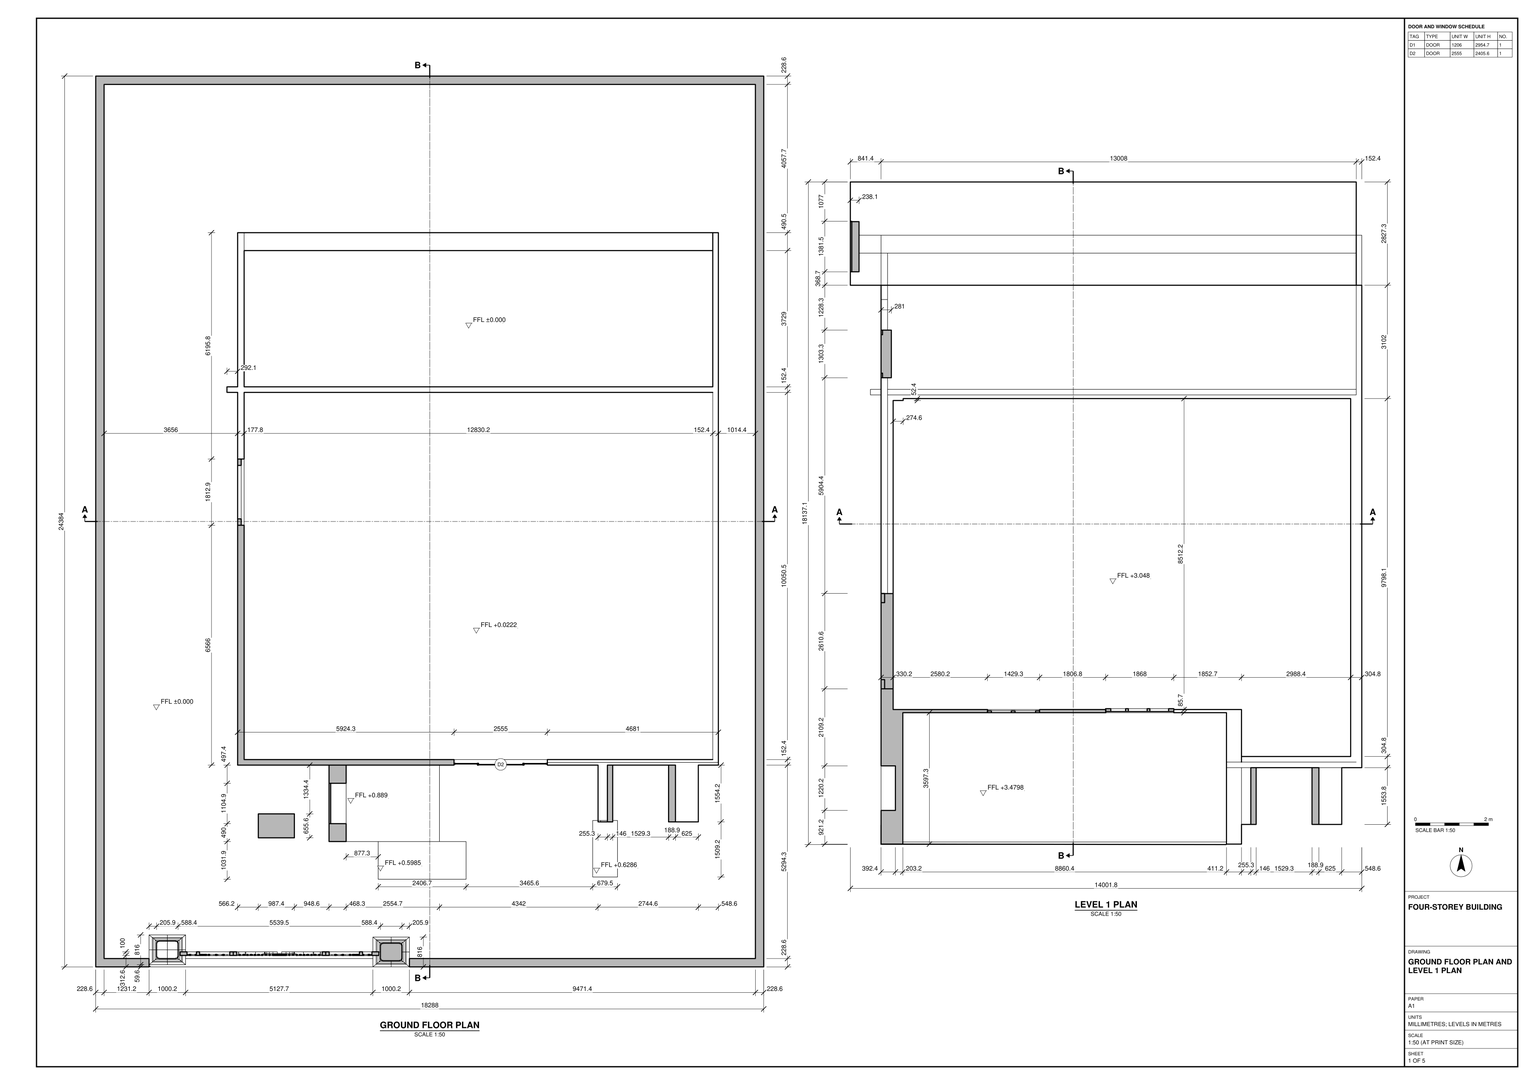
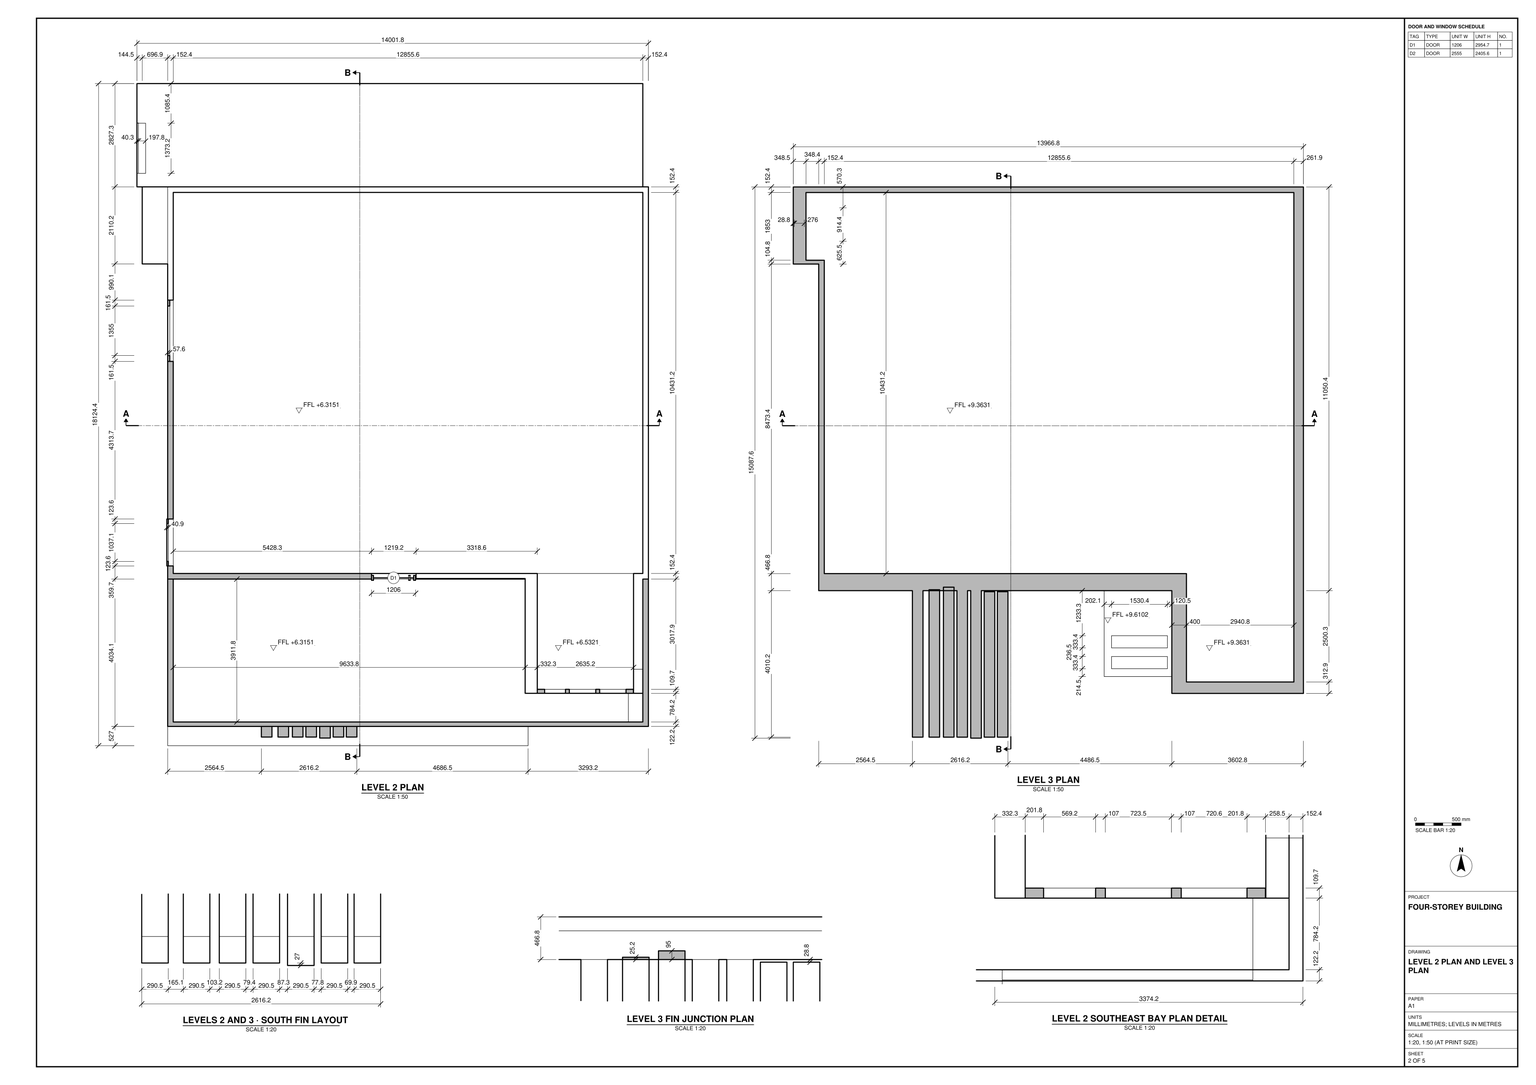
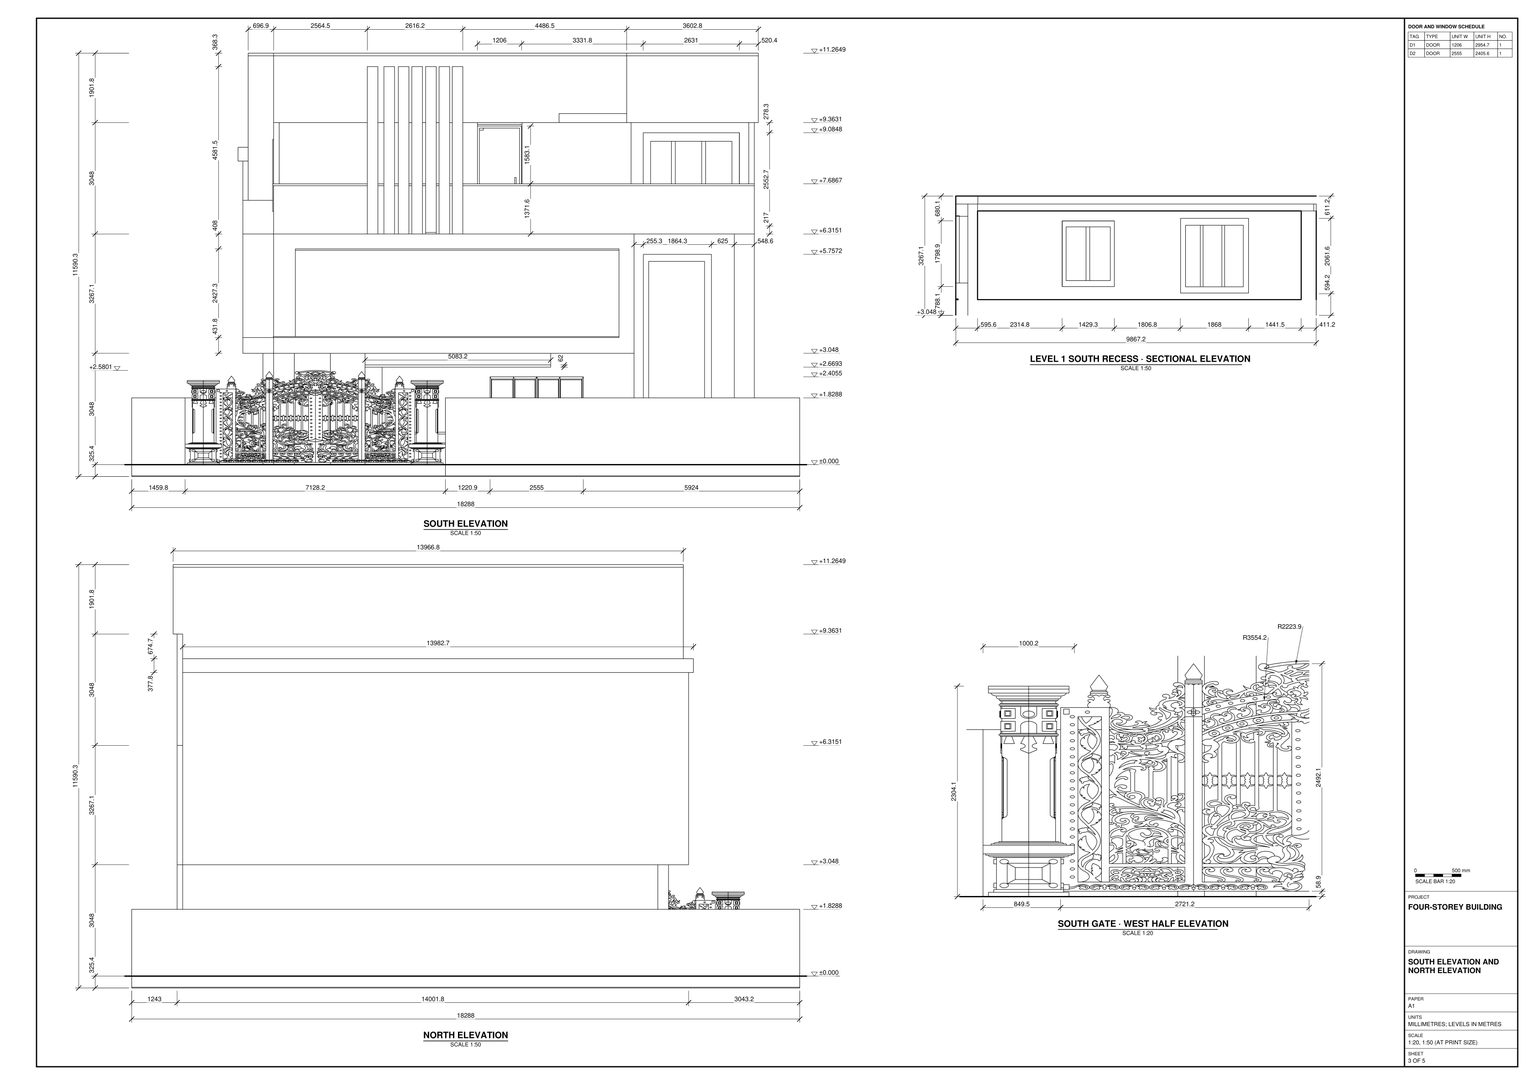
Build the four-storey building and its enclosed site in SketchUp from task_files/diagram_01.pdf. Work in millimetres. The complete model, including the site, measures 18288 mm east–west, 24384 mm north–south and 11590.3 mm from bottom to top. Set the ground floor at 0 mm and the successive storey levels at +3048 mm, +6315.1 mm and +9363.1 mm. Keep the local changes in slab height shown on the plans distinct from these storey levels.

Set out the perimeter wall, the gate and its flanking piers on the south boundary. Position the building within the enclosure using the setbacks on the ground-floor plan. Follow the wall thicknesses and slab edges on each plan rather than repeating one footprint through all four storeys. Model the flat roof and parapets, the projecting bays, and the doors and windows in their drawn openings. Use the sectional elevation to place the windows behind the frame of the Level 1 south recess. Above it, use the plan details to set out the vertical fins and the glazed southeast bay.

Keep shell elements such as walls, slabs and roof, and each furniture or joinery piece shown, in separate groups or components. Use components for repeated parts. Decor and loose items may be any suitable library components. Save one SketchUp model as output_files/four_storey_building_and_its_gated_enclosure.skp.

# SketchUp Ruby script. Lengths in millimetres.
U = 1.mm
M = Sketchup.active_model
def pt(a) = Geom::Point3d.new(a.map { |v| v * U })
def face(e, loops, mat)
  f = e.add_face(loops[0].map { |a| pt(a) })
  loops[1..].each { |l| e.add_face(l.map { |a| pt(a) }).erase! }
  f.material = f.back_material = mat if mat
  f
end
# faces: each face lists its corners as indices into pts; further lists are holes
def faces(e, pts, list, mat = nil) = list.each { |f| face(e, (f[0].is_a?(Array) ? f : [f]).map { |l| l.map { |i| pts[i] } }, mat) }
# xy, xz, yz: faces in a plane at the given z, y or x. An outline is a flat list of corners, or four numbers for a rectangle; further outlines are holes
def ring(l) = l.size == 4 ? [[l[0], l[1]], [l[2], l[1]], [l[2], l[3]], [l[0], l[3]]] : l.each_slice(2).to_a
def flat(e, list, mat, &to3) = list.each { |f| face(e, (f[0].is_a?(Array) ? f : [f]).map { |l| ring(l).map { |u, v| to3.(u, v) } }, mat) }
def xy(e, z, list, mat = nil) = flat(e, list, mat) { |x, y| [x, y, z] }
def xz(e, y, list, mat = nil) = flat(e, list, mat) { |x, z| [x, y, z] }
def yz(e, x, list, mat = nil) = flat(e, list, mat) { |y, z| [x, y, z] }
def lines(e, pts, list) = list.each { |a, b| e.add_line(pt(pts[a]), pt(pts[b])) }
# prism: a flat outline (further loops are holes) pulled along v
def prism(e, loops, v, mat = nil)
  f = face(e, loops, mat); d = Geom::Vector3d.new(v.map { |x| x * U })
  f.pushpull(f.normal.samedirection?(d) ? d.length : -d.length)
end
def box(e, o, s, mat = nil) = prism(e, [[o, [o[0] + s[0], o[1], o[2]], [o[0] + s[0], o[1] + s[1], o[2]], [o[0], o[1] + s[1], o[2]]]], [0, 0, s[2]], mat)
def at(x, y, z, deg = 0) = Geom::Transformation.translation(pt([x, y, z])) * Geom::Transformation.rotation(ORIGIN, Z_AXIS, deg.degrees)
def axes(o, x, y, z) = Geom::Transformation.new([*x, 0, *y, 0, *z, 0, *pt(o).to_a, 1])
def part(name) = M.definitions.add(name)
# library, detail: a bought-in or finely detailed component or shape, given as its bounding box
def library(name, o, s) = part(name).tap { |d| box(d.entities, o, s) }
def detail(e, o, s) = box(e.add_group.entities, o, s)
def put(e, d, t, mat = nil) = e.add_instance(d, t).tap { |i| i.material = mat if mat }
def group(e, t, mat = nil) = e.add_group.tap { |g| g.transformation = t; g.material = mat if mat }.entities
root = M.entities
M.materials.add("[0128_White]").color = [255, 255, 255]
M.materials.add("[Color C08]").color = [102, 51, 0]
M.materials.add("[Color D02]").color = [255, 229, 153]
M.materials.add("[Color M04]").color = [188, 188, 188]
M.materials.add("[Color M06]").color = [86, 86, 86]
M.materials.add("[Color M07]").color = [58, 58, 58]
M.materials.add("[Color M07]1").color = [58, 58, 58]
M.materials.add("[Concrete Scored Jointless]").color = [140, 133, 127]
M.materials.add("[Metal_Corrogated_Shiny]").color = [193, 193, 193]
M.materials.add("[Translucent Glass Blue]").color = [100, 149, 237]
M.materials["[Translucent Glass Blue]"].alpha = 0.5
M.materials.add("[Translucent Glass Gray]").color = [128, 128, 128]
M.materials["[Translucent Glass Gray]"].alpha = 0.5
M.materials.add("[Wood Fence with Lattice]").color = [170, 106, 61]
M.materials.add("[Wood OSB]").color = [240, 195, 122]
M.materials.add("[Wood Veneer 01]").color = [120, 70, 37]
c1 = part("Component\#1")
box(c1.entities,[0,0,0],[8,40,80],"[Metal_Corrogated_Shiny]")
c2 = part("Door pull handle")
prism(c2.entities,[[[0,30,890],[0,30,900],[50,30,900],[50,30,0],[0,30,0],[0,30,10],[40,30,10],[40,30,890]]],[0,-30,0],"[Color M07]")
c3 = part("Framed glass door")
g1 = group(c3.entities,at(41,40,0))
g2 = group(g1,at(-46,0,0))
g3 = group(g2,at(45,0,0))
p = [[15,0,2060],[15,820,2060]]
lines(g3,p,[[0,1]])
g4 = group(g3,at(15,0,0))
yz(g4,0,[[0,0,820,2060]],"[Translucent Glass Gray]")
g5 = group(g2,at(-48.3,0,0))
put(g5,c1,axes([104.3,0,2060],[1,0,0],[0,0,-1],[0,1,0]))
put(g5,c1,axes([104.3,0,40],[1,0,0],[0,0,-1],[0,1,0]))
g6 = group(g2,at(0,720,200))
put(g6,c2,axes([60,0,0],[-1,0,0],[0,1,0],[0,0,1]))
put(g6,c2,at(60,0,0))
g7 = group(c3.entities,at(105,0,0))
g8 = group(g7,at(-100,0,0))
prism(g8,[[[100,860,0],[100,900,0],[100,900,2100],[100,0,2100],[100,0,0],[100,40,0],[100,40,2060],[100,860,2060]]],[-100,0,0],"[Metal_Corrogated_Shiny]")
c4 = part("door glass")
put(c4.entities,c3,at(0,105,0,-90))
c5 = library("20170416 - Larg Glass Door",[-30,0,0],[170,4000,2000])
c6 = library("Gate pier",[0,0,0],[850,850,3692.5])
c7 = library("Drawing1.dwg",[3859.7,90,-250],[4440,3834.1,108])
c8 = part("cổng")
p = [[0,0,0],[25.4,0,0],[492,0,0],[25.4,25.4,0]]
lines(c8.entities,p,[[0,1],[1,2],[1,3],[3,0]])
put(c8.entities,c6,axes([0,59.6,0.7],[0.96,0,0],[0,0.96,0],[0,0,0.96]),"[0128_White]")
put(c8.entities,c6,axes([4999.3,0,0],[0.96,0,0],[0,0.96,0],[0,0,0.96]),"[0128_White]")
put(c8.entities,c7,axes([-3166.7,162.6,0.7],[1,0,0],[0,0,1],[0,-1,0]),"[Color M04]")
g9 = group(c8.entities,at(2510.2,307.6,3835.3),"[Color M07]1")
prism(g9,[[[36.5,5,67.1],[0,5,7.2],[51.1,5,24.7],[108.8,5,44.6],[166.3,5,60.6],[224.7,5,73.1],[283.7,5,82.1],[343.2,5,87.5],[402.9,5,89.3],[462.5,5,87.5],[522,5,82.1],[581,5,73.1],[639.4,5,60.6],[696.9,5,44.6],[754.7,5,24.7],[826.5,5,0],[769.2,5,67.1],[710.2,5,87.4],[650.1,5,104.1],[589.1,5,117.2],[527.4,5,126.5],[465.2,5,132.2],[402.9,5,134.1],[340.5,5,132.2],[278.3,5,126.5],[216.6,5,117.2],[155.6,5,104.1],[95.5,5,87.4]]],[0,25,0])
c9 = part("Group\#1")
xy(c9.entities,0,[[0,0,152.4,862]])
xy(c9.entities,83,[[0,83,152.4,779]],"[Color C08]")
xy(c9.entities,779,[[0,83,152.4,779]],"[Color C08]")
xy(c9.entities,862,[[0,0,152.4,862]],"[Color C08]")
xz(c9.entities,0,[[0,0,152.4,862]],"[Color C08]")
xz(c9.entities,83,[[0,83,152.4,779]],"[Color C08]")
xz(c9.entities,779,[[0,83,152.4,779]],"[Color C08]")
xz(c9.entities,862,[[0,0,152.4,862]],"[Color C08]")
yz(c9.entities,0,[[[0,0,862,862],[83,83,779,779]]],"[Color C08]")
yz(c9.entities,0,[[83,83,779,779]],"[Translucent Glass Gray]")
yz(c9.entities,152.4,[[[0,0,862,862],[83,83,779,779]]],"[Color C08]")
c10 = part("Group\#2")
xy(c10.entities,0,[[0,0,3233.7,152.4]])
xy(c10.entities,248.1,[[1480.7,0,1712.7,152.4]])
xy(c10.entities,248.1,[[248.1,0,1480.7,152.4],[1712.7,0,2985.7,152.4]],"[Color C08]")
xy(c10.entities,2469.7,[[248.1,0,1480.7,152.4],[1480.7,0,1712.7,152.4],[1712.7,0,2985.7,152.4]])
xy(c10.entities,2717.8,[[0,0,3233.7,152.4]],"[Color C08]")
xz(c10.entities,0,[[[0,0,3233.7,2717.8],[248.1,248.1,2985.7,2469.7]],[1480.7,248.1,1712.7,2469.7]],"[Color C08]")
xz(c10.entities,0,[[248.1,248.1,1480.7,2469.7],[1712.7,248.1,2985.7,2469.7]],"[Translucent Glass Gray]")
xz(c10.entities,152.4,[[[0,0,3233.7,2717.8],[248.1,248.1,2985.7,2469.7]],[1480.7,248.1,1712.7,2469.7]],"[Color C08]")
yz(c10.entities,0,[[0,0,152.4,2717.8]],"[Color C08]")
yz(c10.entities,248.1,[[0,248.1,152.4,2469.7]],"[Color C08]")
yz(c10.entities,1480.7,[[0,248.1,152.4,2469.7]],"[Color C08]")
yz(c10.entities,1712.7,[[0,248.1,152.4,2469.7]],"[Color C08]")
yz(c10.entities,2985.7,[[0,248.1,152.4,2469.7]],"[Color C08]")
yz(c10.entities,3233.7,[[0,0,152.4,2717.8]],"[Color C08]")
c11 = part("Group\#3")
xy(c11.entities,0,[[0,0,3233.7,152.4]])
xy(c11.entities,248.1,[[947.7,0,1079.2,152.4],[1968.5,0,2100,152.4]])
xy(c11.entities,248.1,[[248.1,0,947.7,152.4],[1079.2,0,1968.5,152.4],[2100,0,2985.7,152.4]],"[Color C08]")
xy(c11.entities,2469.7,[[248.1,0,947.7,152.4],[947.7,0,1079.2,152.4],[1079.2,0,1968.5,152.4],[1968.5,0,2100,152.4],[2100,0,2985.7,152.4]])
xy(c11.entities,2717.8,[[0,0,3233.7,152.4]],"[Color C08]")
xz(c11.entities,0,[[[0,0,3233.7,2717.8],[248.1,248.1,2985.7,2469.7]],[947.7,248.1,1079.2,2469.7],[1968.5,248.1,2100,2469.7]],"[Color C08]")
xz(c11.entities,0,[[248.1,248.1,947.7,2469.7],[1079.2,248.1,1968.5,2469.7],[2100,248.1,2985.7,2469.7]],"[Translucent Glass Gray]")
xz(c11.entities,152.4,[[[0,0,3233.7,2717.8],[248.1,248.1,2985.7,2469.7]],[947.7,248.1,1079.2,2469.7],[1968.5,248.1,2100,2469.7]],"[Color C08]")
yz(c11.entities,0,[[0,0,152.4,2717.8]],"[Color C08]")
yz(c11.entities,248.1,[[0,248.1,152.4,2469.7]],"[Color C08]")
yz(c11.entities,947.7,[[0,248.1,152.4,2469.7]],"[Color C08]")
yz(c11.entities,1079.2,[[0,248.1,152.4,2469.7]],"[Color C08]")
yz(c11.entities,1968.5,[[0,248.1,152.4,2469.7]],"[Color C08]")
yz(c11.entities,2100,[[0,248.1,152.4,2469.7]],"[Color C08]")
yz(c11.entities,2985.7,[[0,248.1,152.4,2469.7]],"[Color C08]")
yz(c11.entities,3233.7,[[0,0,152.4,2717.8]],"[Color C08]")
xy(root,-20.6,[[0,0,18288,24384]])
xy(root,0,[[0,0,18288,24384]])
xy(root,304.8,[[1459.8,0,8588,228.6],[6386.8,3430.6,9409.8,5522.9],[15871.3,3968.7,16496.3,3968.7,16496.3,5522.9,17045,5522.9,17045,5597.5,12363.9,5597.5,12363.9,5522.9,13751.8,5522.9,13751.8,4007.4,14007,4007.4,14007,5522.9,15871.3,5522.9],[13751.8,3968.7,13821.3,4007.4],[15682.4,3968.7,15871.3,5522.9],
  [14007,4007.4,14153.1,5522.9],[5844.3,5522.9,8644.6,5522.9,8644.6,5597.5,9808.9,5597.5,9808.9,5675.3,4062.4,5675.3,4062.4,15725.8,16892.6,15725.8,16892.6,5675.3,12363.9,5675.3,12363.9,5597.5,17045,5597.5,17045,20097.7,16892.6,20097.7,16892.6,15878.2,4062.4,15878.2,4062.4,20097.7,3884.6,20097.7,3884.6,15878.2,3592.5,15878.2,3592.5,15725.8,3884.6,15725.8,3884.6,5597.5,5844.3,5597.5],[3884.6,5522.9,5844.3,5597.5],[8644.6,5522.9,9808.9,5597.5],[4062.4,15878.2,16892.6,19607.2],
  [4062.4,19607.2,16892.6,20097.7]])
xy(root,304.8,[[[228.6,228.6,18059.4,24155.4],[7732.5,2398.7,7732.5,3430.6,6386.8,3430.6,6386.8,5522.9,3884.6,5522.9,3884.6,15725.8,3592.5,15725.8,3592.5,15878.2,3884.6,15878.2,3884.6,20097.7,17045,20097.7,17045,5522.9,16496.3,5522.9,16496.3,3968.7,15682.4,3968.7,15682.4,5522.9,14153.1,5522.9,14153.1,4007.4,14284.1,4007.4,14284.1,2459.6,13604.7,2459.6,13604.7,4007.4,13751.8,4007.4,13751.8,5522.9,12363.9,5522.9,12363.9,5675.3,9808.9,5675.3,9808.9,5522.9,9409.8,5522.9,9409.8,3430.6,10139.1,3430.6,10139.1,2398.7],[4450.8,3532.8,5438.2,4188.5]]],"[Concrete Scored Jointless]")
xy(root,304.8,[[0,0,0,24384,18288,24384,18288,0,8588,0,8588,228.6,18059.4,228.6,18059.4,24155.4,228.6,24155.4,228.6,228.6,1459.8,228.6,1459.8,0]],"[Wood Fence with Lattice]")
xy(root,327,[[4062.4,5675.3,16892.6,15725.8]])
xy(root,858.8,[[7732.5,2398.7,10139.1,3430.6],[13604.7,2459.6,13604.7,4007.4,13751.8,4007.4,13751.8,3968.7,13821.3,3968.7,13821.3,4007.4,14284.1,4007.4,14284.1,2459.6]])
xy(root,903.3,[[7732.5,2398.7,10139.1,3430.6]],"[Color M06]")
xy(root,933.4,[[13821.3,3968.7,14007,4007.4],[14007,3968.7,14153.1,4007.4]])
xy(root,933.4,[[13604.7,2459.6,14284.1,2459.6,14284.1,4007.4,14153.1,4007.4,14153.1,3968.7,13751.8,3968.7,13751.8,4007.4,13604.7,4007.4]],"[Color M06]")
xy(root,1143,[[6386.8,3430.6,9409.8,5522.9]])
xy(root,1193.8,[[6386.8,3430.6,6855.1,5522.9]])
xy(root,1193.8,[[6855.1,3430.6,9409.8,5522.9]],"[Color M06]")
xy(root,1197.6,[[3884.6,12089,4062.4,13901.9]])
xy(root,1449.5,[[6386.8,3920.6,6855.1,5025.5]])
xy(root,2133.6,[[0,0,1459.8,0,1459.8,228.6,228.6,228.6,228.6,24155.4,18059.4,24155.4,18059.4,228.6,8588,228.6,8588,0,18288,0,18288,24384,0,24384]],"[Wood Fence with Lattice]")
xy(root,2225,[[3884.6,7579.3,4062.4,8200],[3884.6,8890.5,4062.4,9511.3]])
xy(root,2603.6,[[6386.8,3920.6,6855.1,5025.5]])
xy(root,2710.4,[[9808.9,5522.9,12363.9,5597.5],[9808.9,5597.5,12363.9,5675.3]])
xy(root,2885.1,[[3884.6,12089,4062.4,13901.9]])
xy(root,2952,[[3884.6,7579.3,4062.4,8200],[3884.6,8890.5,4062.4,9511.3]])
xy(root,2974.1,[[6386.8,3430.6,6855.1,3743.8],[6855.1,3430.6,11470,3743.8],[6386.8,3743.8,6855.1,5522.9]])
xy(root,3352.8,[[3884.6,3430.6,6386.8,5522.9],[6386.8,3430.6,6855.1,5522.9],[6855.1,3430.6,11470,3743.8],[4450.8,3532.8,5438.2,4188.5],[13751.8,5827.7,16740.2,5827.7,16740.2,15625.8,4489.5,15625.8,4489.5,15573.4,4214.8,15573.4,4214.8,7113.6,13751.8,7113.6],
  [3592.5,15725.8,3884.6,15878.2],[4062.4,15725.8,16892.6,15878.2],[4062.4,15878.2,16892.6,18727.7],[3884.6,18337.2,4062.4,18727.7],[3043.2,18727.7,3884.6,19607.2],
  [3884.6,18727.7,4062.4,19607.2],[16892.6,18727.7,17045,20097.7],[3043.2,19607.2,3884.6,20097.7],[3884.6,19607.2,16892.6,20097.7],[3043.2,20097.7,16892.6,21555]])
xy(root,3352.8,[[11470,3430.6,11470,3743.8,6855.1,3743.8,6855.1,5522.9,13751.8,5522.9,13751.8,3430.6]],"[Color M06]")
xy(root,3784.6,[[3884.6,3417.9,13340.6,3430.6],[3884.6,3430.6,3884.6,7027.9,3946.9,7027.9,3946.9,3488.3,13340.6,3488.3,13340.6,3430.6],[4480.2,3488.3,13340.6,7027.9],[3884.6,7027.9,3946.9,8570.9]])
xy(root,3797.3,[[3884.6,3954.9,3946.9,4215.3],[3884.6,4215.3,3946.9,5927.6],[3884.6,5927.6,3946.9,7027.9]])
xy(root,3810,[[3875.1,3417.9,13340.6,3417.9,4480.2,3430.6,3884.6,3430.6,3884.6,3954.9,3875.1,3954.9],[13340.6,3417.9,13340.6,3488.3,4480.2,3488.3,4480.2,3430.6],[3884.6,3430.6,3946.9,3954.9],[3946.9,3430.6,4480.2,3488.3],[3884.6,7027.9,3946.9,8570.9]])
xy(root,3964,[[10038.6,7027.9,11899.1,7113.6]])
xy(root,4140.9,[[6800.3,7027.9,8224.3,7113.6]])
xy(root,4238.9,[[3884.6,7681.2,4214.8,10287.8]])
xy(root,4311.6,[[3884.6,4351.8,4277,5572],[4277,4351.8,4287.9,5572]],"[Color D02]")
xy(root,4374.6,[[3043.2,19096.5,3281.4,20469.6]])
xy(root,4378.5,[[3884.6,16196.1,4165.6,17499.5]])
xy(root,5352.9,[[3884.6,14095.4,4214.8,14805]])
xy(root,5869.9,[[14153.1,3968.7,15682.4,5522.9]])
xy(root,5896.4,[[3884.6,4351.8,4277,5572]])
xy(root,5916.8,[[3884.6,16196.1,4165.6,17499.5]])
xy(root,5936.4,[[6800.3,7027.9,8224.3,7113.6]])
xy(root,6008.7,[[10038.6,7027.9,11899.1,7113.6]])
xy(root,6062,[[14007,3968.7,15871.3,5522.9]])
xy(root,6062.5,[[3884.6,14095.4,4214.8,14805]])
xy(root,6064.5,[[3884.6,7681.2,4214.8,10287.8]])
xy(root,6211.9,[[4480.2,3430.6,13340.6,7027.9],[13340.6,5827.7,13685.1,7027.9]])
xy(root,6400.8,[[13751.8,5827.7,13751.8,7113.6,4214.8,7113.6,4214.8,15573.4,16740.2,15573.4,16740.2,5827.7],[4489.5,15573.4,16740.2,15625.8]])
xy(root,6444.7,[[3043.2,19096.5,3281.4,20469.6]])
xy(root,6619.9,[[6449.1,3667.1,6739.6,3957.6],[6904.7,3667.1,7195.2,3957.6],[7298.4,3667.1,7588.9,3957.6],[7668.3,3667.1,7958.8,3957.6],[8046.1,3667.1,8336.6,3957.6],
  [8414.4,3667.1,8704.9,3957.6],[8774.8,3667.1,9065.3,3957.6],[3884.6,3957.6,3884.6,7991.7,4037,7991.7,4037,4079.9,13751.8,4079.9,13751.8,3957.6],[13751.8,3957.6,16496.3,3968.7],[16496.3,3957.6,16496.3,4079.9,16892.6,4079.9,16892.6,5522.9,17045,5522.9,17045,3957.6],
  [13751.8,3968.7,16496.3,4079.9],[4037,4079.9,16496.3,4079.9,16496.3,4864.1,13670.8,4864.1,13670.8,7991.7,4037,7991.7],[16496.3,4079.9,16892.6,4864.1],[13670.8,4864.1,13670.8,8006,10684.5,8006,10684.5,8144.1,16892.6,8144.1,16892.6,18575.3,4037,18575.3,4037,8144.1,9465.3,8144.1,9465.3,7991.7,3884.6,7991.7,3884.6,18727.7,17045,18727.7,17045,7991.7,16892.6,7991.7,16892.6,5522.9,16496.3,5522.9,16496.3,4864.1],[16496.3,4864.1,16892.6,5522.9],
  [16892.6,5522.9,17045,7991.7],[9465.3,7991.7,10684.5,8144.1],[10684.5,7991.7,13670.8,8006],[4037,8144.1,16892.6,18575.3]])
xy(root,6619.9,[[3884.6,3430.6,13751.8,3430.6,13751.8,3957.6,9065.3,3957.6,9065.3,3667.1,8774.8,3667.1,8774.8,3957.6,8704.9,3957.6,8704.9,3667.1,8414.4,3667.1,8414.4,3957.6,8336.6,3957.6,8336.6,3667.1,8046.1,3667.1,8046.1,3957.6,7958.8,3957.6,7958.8,3667.1,7668.3,3667.1,7668.3,3957.6,7588.9,3957.6,7588.9,3667.1,7298.4,3667.1,7298.4,3957.6,7195.2,3957.6,7195.2,3667.1,6904.7,3667.1,6904.7,3957.6,6739.6,3957.6,6739.6,3667.1,6449.1,3667.1,6449.1,3957.6,3884.6,3957.6]],"[Color M06]")
xy(root,6661.2,[[8046.1,3640.1,8336.6,3667.1],[8046.1,3667.1,8336.6,3957.6]])
xy(root,6836.9,[[14003.1,4864.1,16638.4,8144.1]])
xy(root,7233.2,[[3884.6,8351.5,4037,9635.7]])
xy(root,7540.6,[[3187.7,16617.5,3884.6,18727.7]])
xy(root,7553.7,[[3884.6,13949.5,4037,15627.5]])
xy(root,7940.7,[[3860.8,3937,3884.6,7991.7],[3884.6,3937,6449.1,3957.6],[3884.6,3957.6,3884.6,7991.7,4037,7991.7,4037,4079.9,16892.6,4079.9,16892.6,7991.7,17045,7991.7,17045,3957.6]])
xy(root,7991.5,[[3860.8,3937,6449.1,3937,6449.1,3957.6,3884.6,3957.6,3884.6,7991.7,3860.8,7991.7],[3884.6,3957.6,17045,3957.6,17045,7991.7,16892.6,7991.7,16892.6,4079.9,4037,4079.9,4037,7991.7,3884.6,7991.7]],"[Color M06]")
xy(root,8243.8,[[3187.7,17243,3492.5,18157.4]])
xy(root,8615.4,[[2909.9,18727.7,3043.2,21618.5],[3043.2,18727.7,16892.6,21555],[3043.2,21555,16892.6,21618.5]])
xy(root,8993.2,[[2909.9,18727.7,16892.6,21618.5]],"[Color M06]")
xy(root,9122.1,[[3884.6,13949.5,4037,15627.5]])
xy(root,9209.6,[[3884.6,8351.5,4037,9635.7]])
xy(root,9389.6,[[14003.1,4864.1,16638.4,8144.1]])
xy(root,9413.8,[[3187.7,17243,3492.5,18157.4]])
xy(root,9617.1,[[4037,8144.1,16892.6,18575.3]])
xy(root,9667.9,[[13551.8,4864.1,13670.8,5177.1],[16892.6,4864.1,17154.5,5177.1],[13951.8,5177.1,16892.6,5177.1,16892.6,18575.3,3536.2,18575.3,3536.2,16722.3,4037,16722.3,4037,8144.1,13951.8,8144.1],[13551.8,5177.1,13670.8,7677.4],[13670.8,5177.1,13951.8,7677.4],
  [16892.6,5177.1,17154.5,7677.4],[[11698.8,5326.3,11698.8,7677.4,10684.5,7677.4,10684.5,7991.7,13658.1,7991.7,13658.1,7677.4,13551.8,7677.4,13551.8,5326.3],[11900.9,6110.7,13431.3,6444.1],[11900.9,5540.8,13431.3,5874.1]],[3884.6,7677.4,4037,7991.7],[4037,7677.4,9465.3,7991.7],[9465.3,7677.4,10684.5,8144.1],
  [13658.1,7677.4,13670.8,7991.7],[13670.8,7677.4,13951.8,7991.7],[16892.6,7677.4,17154.5,7991.7],[10684.5,7991.7,13658.1,8006],[13658.1,7991.7,13670.8,8006],
  [13670.8,7991.7,13670.8,8006,13658.1,8006,13658.1,8144.1,13951.8,8144.1,13951.8,7991.7],[17045,7991.7,17154.5,18727.7]])
xy(root,9915,[[[11698.8,5326.3,13551.8,7677.4],[11900.9,5540.8,13431.3,5874.1],[11900.9,6110.7,13431.3,6444.1]]])
xy(root,10819.3,[[6449.1,3957.6,6739.6,7677.4],[6904.7,3957.6,7195.2,7702.5],[7298.4,3957.6,7588.9,7772.4],[7668.3,3957.6,7958.8,7677.4],[8046.1,3957.6,8336.6,7677.4],
  [8414.4,3957.6,8704.9,7648.6],[8774.8,3957.6,9065.3,7648.6]])
xy(root,11201.4,[[8046.1,3640.1,8336.6,7677.4],[6449.1,3667.1,6739.6,7677.4],[6904.7,3667.1,7195.2,7702.5],[7298.4,3667.1,7588.9,7772.4],[7668.3,3667.1,7958.8,7677.4],
  [8414.4,3667.1,8704.9,7648.6],[8774.8,3667.1,9065.3,7648.6]])
xy(root,11496.7,[[[13551.8,4864.1,13551.8,7677.4,3884.6,7677.4,3884.6,16617.5,3187.7,16617.5,3187.7,18727.7,17154.5,18727.7,17154.5,4864.1],[13951.8,5177.1,16892.6,5177.1,16892.6,18575.3,3536.2,18575.3,3536.2,16722.3,4037,16722.3,4037,8144.1,13951.8,8144.1]]])
xy(root,11569.7,[[[13551.8,4864.1,17154.5,4864.1,17154.5,18727.7,3187.7,18727.7,3187.7,16617.5,3884.6,16617.5,3884.6,7677.4,13551.8,7677.4],[13951.8,5177.1,13951.8,8144.1,4037,8144.1,4037,16722.3,3536.2,16722.3,3536.2,18575.3,16892.6,18575.3,16892.6,5177.1]]],"[Color M06]")
xz(root,0,[[0,-20.6,18288,0]])
xz(root,0,[[0,0,8588,304.8],[8588,0,18288,304.8],[0,304.8,1459.8,2133.6],[8588,304.8,18288,2133.6]],"[Wood Fence with Lattice]")
xz(root,228.6,[[228.6,304.8,1459.8,2133.6],[8588,304.8,18059.4,2133.6]],"[Wood Fence with Lattice]")
xz(root,2398.7,[[7732.5,858.8,10139.1,903.3]],"[Color M06]")
xz(root,2398.7,[[7732.5,304.8,10139.1,858.8]],"[Wood OSB]")
xz(root,2459.6,[[13604.7,858.8,14284.1,933.4]],"[Color M06]")
xz(root,2459.6,[[13604.7,304.8,14284.1,858.8]],"[Wood OSB]")
xz(root,3417.9,[[3875.1,3784.6,13340.6,3810]])
xz(root,3430.6,[[7732.5,304.8,9409.8,858.8],[9409.8,304.8,10139.1,858.8],[7732.5,858.8,9409.8,903.3],[9409.8,858.8,10139.1,903.3],[6386.8,1193.8,6855.1,2974.1]])
xz(root,3430.6,[[6386.8,1143,9409.8,1193.8],[6386.8,2974.1,11470,3036.1],[6386.8,3036.1,11470,3352.8],[3884.6,3352.8,13751.8,3352.8,13751.8,6619.9,3884.6,6619.9,3884.6,3810,4480.2,3810,4480.2,6211.9,13340.6,6211.9,13340.6,3784.6,3884.6,3784.6]],"[Color M06]")
xz(root,3430.6,[[6386.8,304.8,7732.5,304.8,7732.5,903.3,9409.8,903.3,9409.8,1143,6386.8,1143]],"[Wood OSB]")
xz(root,3488.3,[[3946.9,3784.6,4480.2,3810],[4480.2,3784.6,13340.6,3810]])
xz(root,3532.8,[[4450.8,304.8,5438.2,3352.8]],"[Color M06]")
xz(root,3640.1,[[8046.1,6661.2,8336.6,11201.4]])
xz(root,3667.1,[[6449.1,6619.9,6739.6,11201.4],[6904.7,6619.9,7195.2,11201.4],[7298.4,6619.9,7588.9,11201.4],[7668.3,6619.9,7958.8,11201.4],[8046.1,6619.9,8336.6,6661.2],
  [8414.4,6619.9,8704.9,11201.4],[8774.8,6619.9,9065.3,11201.4]])
xz(root,3743.8,[[6855.1,2974.1,11470,3352.8]],"[Color M06]")
xz(root,3920.6,[[6386.8,1449.5,6855.1,2603.6]])
xz(root,3937,[[3860.8,7940.7,6449.1,7991.5]],"[Color M06]")
xz(root,3954.9,[[3884.6,3797.3,3946.9,3810]])
xz(root,3957.6,[[6449.1,6619.9,6739.6,7940.7],[6739.6,6619.9,6904.7,7940.7],[6904.7,6619.9,7195.2,7940.7],[7195.2,6619.9,7298.4,7940.7],[7298.4,6619.9,7588.9,7940.7],
  [7588.9,6619.9,7668.3,7940.7],[7668.3,6619.9,7958.8,7940.7],[7958.8,6619.9,8046.1,7940.7],[8046.1,6619.9,8336.6,6661.2],[8336.6,6619.9,8414.4,7940.7],
  [8414.4,6619.9,8704.9,7940.7],[8704.9,6619.9,8774.8,7940.7],[8774.8,6619.9,9065.3,7940.7],[8046.1,6661.2,8336.6,7940.7],[3884.6,7940.7,6449.1,7991.5],
  [6449.1,7940.7,6739.6,7991.5],[6739.6,7940.7,6904.7,7991.5],[6904.7,7940.7,7195.2,7991.5],[7195.2,7940.7,7298.4,7991.5],[7298.4,7940.7,7588.9,7991.5],
  [7588.9,7940.7,7668.3,7991.5],[7668.3,7940.7,7958.8,7991.5],[7958.8,7940.7,8046.1,7991.5],[8046.1,7940.7,8336.6,7991.5],[8336.6,7940.7,8414.4,7991.5],
  [8414.4,7940.7,8704.9,7991.5],[8704.9,7940.7,8774.8,7991.5],[8774.8,7940.7,9065.3,7991.5],[6449.1,7991.5,6739.6,10819.3],[6904.7,7991.5,7195.2,10819.3],
  [7298.4,7991.5,7588.9,10819.3],[7668.3,7991.5,7958.8,10819.3],[8046.1,7991.5,8336.6,10819.3],[8414.4,7991.5,8704.9,10819.3],[8774.8,7991.5,9065.3,10819.3]])
xz(root,3957.6,[[9065.3,7940.7,17045,7991.5]],"[Color M06]")
xz(root,3957.6,[[3884.6,6619.9,6449.1,7940.7],[9065.3,6619.9,17045,7940.7]],"[Translucent Glass Blue]")
xz(root,3968.7,[[13751.8,304.8,13821.3,858.8],[15871.3,304.8,16496.3,304.8,16496.3,6619.9,13751.8,6619.9,13751.8,933.4,14007,933.4,14007,6062,15871.3,6062],[13751.8,858.8,13821.3,933.4]])
xz(root,3968.7,[[15682.4,304.8,15871.3,304.8,15871.3,6062,14007,6062,14007,933.4,14153.1,933.4,14153.1,5869.9,15682.4,5869.9]],"[Wood Veneer 01]")
xz(root,4007.4,[[13821.3,304.8,14007,858.8],[14007,304.8,14153.1,858.8],[13821.3,858.8,14007,933.4],[14007,858.8,14153.1,933.4]])
xz(root,4007.4,[[13604.7,858.8,13751.8,933.4],[14153.1,858.8,14284.1,933.4]],"[Color M06]")
xz(root,4007.4,[[13604.7,304.8,13751.8,858.8],[14153.1,304.8,14284.1,858.8]],"[Wood OSB]")
xz(root,4079.9,[[4037,7940.7,16892.6,7991.5]],"[Color M06]")
xz(root,4079.9,[[4037,6619.9,16892.6,7940.7]],"[Translucent Glass Blue]")
xz(root,4188.5,[[4450.8,304.8,5438.2,3352.8]],"[Color M06]")
xz(root,4351.8,[[3884.6,4311.6,4277,5896.4]],"[Color D02]")
xz(root,4864.1,[[[13670.8,6619.9,16892.6,9667.9],[14003.1,6836.9,16638.4,9389.6]],[13551.8,9667.9,17154.5,11496.7]])
xz(root,4864.1,[[13551.8,11496.7,17154.5,11569.7]],"[Color M06]")
xz(root,5025.5,[[6386.8,1449.5,6855.1,2603.6]])
xz(root,5177.1,[[13951.8,9667.9,16892.6,11496.7]])
xz(root,5177.1,[[13951.8,11496.7,16892.6,11569.7]],"[Color M06]")
xz(root,5326.3,[[11698.8,9667.9,13551.8,9915]])
xz(root,5522.9,[[3884.6,304.8,6386.8,3352.8],[6386.8,304.8,8644.6,1143],[9409.8,304.8,9808.9,304.8,9808.9,2710.4,12363.9,2710.4,12363.9,304.8,13751.8,304.8,13751.8,3352.8,6855.1,3352.8,6855.1,1193.8,9409.8,1193.8],[8644.6,304.8,9409.8,1143],[14007,304.8,14153.1,3352.8],
  [15682.4,304.8,15871.3,3352.8],[16496.3,304.8,17045,6619.9],[6386.8,1143,9409.8,1193.8],[6386.8,1193.8,6855.1,2974.1],[6386.8,2974.1,6855.1,3352.8],
  [14007,3352.8,14153.1,5869.9],[15682.4,3352.8,15871.3,5869.9],[14007,5869.9,15871.3,6062]])
xz(root,5522.9,[[14153.1,304.8,15682.4,5869.9]],"[Wood Veneer 01]")
xz(root,5540.8,[[11900.9,9667.9,13431.3,9915]])
xz(root,5572,[[3884.6,4311.6,4277,5896.4]],"[Color D02]")
xz(root,5675.3,[[4062.4,304.8,9808.9,327],[9808.9,304.8,12363.9,327],[12363.9,304.8,16892.6,327],[4062.4,327,4062.4,3352.8,16892.6,3352.8,16892.6,327,12363.9,327,12363.9,2710.4,9808.9,2710.4,9808.9,327]])
xz(root,5827.7,[[13751.8,3352.8,16740.2,6400.8],[13685.1,6211.9,13751.8,6400.8]])
xz(root,5874.1,[[11900.9,9667.9,13431.3,9915]])
xz(root,6110.7,[[11900.9,9667.9,13431.3,9915]])
xz(root,6444.1,[[11900.9,9667.9,13431.3,9915]])
xz(root,7027.9,[[3884.6,3784.6,3946.9,3797.3],[3884.6,3797.3,3946.9,3810],[4480.2,6211.9,13685.1,6400.8]])
xz(root,7027.9,[[[4480.2,3784.6,13340.6,6211.9],[10038.6,3964,11899.1,6008.7],[6800.3,4140.9,8224.3,5936.4]]],"[Color D02]")
xz(root,7113.6,[[[4214.8,3352.8,13751.8,6400.8],[10038.6,3964,11899.1,6008.7],[6800.3,4140.9,8224.3,5936.4]]])
xz(root,7579.3,[[3884.6,2225,4062.4,2952]])
xz(root,7648.6,[[8414.4,10819.3,8704.9,11201.4],[8774.8,10819.3,9065.3,11201.4]])
xz(root,7677.4,[[[3884.6,9667.9,11698.8,9667.9,11698.8,9915,13551.8,9915,13551.8,11496.7,3884.6,11496.7],[8046.1,10819.3,8336.6,11201.4],[6449.1,10819.3,6739.6,11201.4],[7668.3,10819.3,7958.8,11201.4]]])
xz(root,7677.4,[[3884.6,11496.7,13551.8,11569.7]],"[Color M06]")
xz(root,7681.2,[[3884.6,4238.9,4214.8,6064.5]])
xz(root,7702.5,[[6904.7,10819.3,7195.2,11201.4]])
xz(root,7772.4,[[7298.4,10819.3,7588.9,11201.4]])
xz(root,7991.7,[[3884.6,6619.9,4037,7940.7],[4037,6619.9,9465.3,9667.9],[10684.5,6619.9,13670.8,9667.9],[16892.6,6619.9,17045,7940.7],[3860.8,7940.7,3884.6,7991.5],
  [3884.6,7940.7,4037,7991.5],[16892.6,7940.7,17045,7991.5],[3884.6,7991.5,4037,9667.9],[16892.6,7991.5,17045,9667.9]])
xz(root,8006,[[10684.5,6619.9,13670.8,9667.9]])
xz(root,8144.1,[[4037,6619.9,9465.3,9617.1],[9465.3,6619.9,10684.5,9617.1],[[10684.5,6619.9,16892.6,9617.1],[14003.1,6836.9,16638.4,9389.6]],[4037,9617.1,9465.3,9667.9],[9465.3,9617.1,10684.5,9667.9],
  [4037,9667.9,13951.8,11496.7]])
xz(root,8144.1,[[4037,11496.7,13951.8,11569.7]],"[Color M06]")
xz(root,8200,[[3884.6,2225,4062.4,2952]])
xz(root,8351.5,[[3884.6,7233.2,4037,9209.6]])
xz(root,8570.9,[[3884.6,3784.6,3946.9,3810]])
xz(root,8890.5,[[3884.6,2225,4062.4,2952]])
xz(root,9511.3,[[3884.6,2225,4062.4,2952]])
xz(root,9635.7,[[3884.6,7233.2,4037,9209.6]])
xz(root,10287.8,[[3884.6,4238.9,4214.8,6064.5]])
xz(root,12089,[[3884.6,1197.6,4062.4,2885.1]])
xz(root,13901.9,[[3884.6,1197.6,4062.4,2885.1]])
xz(root,13949.5,[[3884.6,7553.7,4037,9122.1]])
xz(root,14095.4,[[3884.6,5352.9,4214.8,6062.5]])
xz(root,14805,[[3884.6,5352.9,4214.8,6062.5]])
xz(root,15573.4,[[4214.8,3352.8,4489.5,6400.8]])
xz(root,15625.8,[[4489.5,3352.8,16740.2,6400.8]])
xz(root,15627.5,[[3884.6,7553.7,4037,9122.1]])
xz(root,15725.8,[[3592.5,304.8,3884.6,3352.8],[4062.4,304.8,16892.6,327],[4062.4,327,16892.6,3352.8]])
xz(root,15878.2,[[3592.5,304.8,3884.6,1175.8],[4062.4,304.8,16892.6,3352.8],[3592.5,1175.8,3884.6,3352.8]])
xz(root,16196.1,[[3884.6,4378.5,4165.6,5916.8]])
xz(root,16617.5,[[3187.7,7540.6,3884.6,11496.7]])
xz(root,16617.5,[[3187.7,11496.7,3884.6,11569.7]],"[Color M06]")
xz(root,16722.3,[[3536.2,9667.9,4037,11496.7]])
xz(root,16722.3,[[3536.2,11496.7,4037,11569.7]],"[Color M06]")
xz(root,17243,[[3187.7,8243.8,3492.5,9413.8]])
xz(root,17499.5,[[3884.6,4378.5,4165.6,5916.8]])
xz(root,18157.4,[[3187.7,8243.8,3492.5,9413.8]])
xz(root,18575.3,[[4037,6619.9,4062.4,9617.1],[4062.4,6619.9,16892.6,9617.1],[4037,9617.1,4062.4,9667.9],[4062.4,9617.1,4398.1,9667.9],[4398.1,9617.1,4658.4,9667.9],
  [4658.4,9617.1,16892.6,9667.9],[3536.2,9667.9,16892.6,11496.7]])
xz(root,18575.3,[[3536.2,11496.7,16892.6,11569.7]],"[Color M06]")
xz(root,18727.7,[[3043.2,3352.8,3884.6,3784.6],[3884.6,3352.8,16892.6,6619.9],[16892.6,3352.8,17045,6619.9],[3043.2,3784.6,3884.6,6619.9],[3043.2,6619.9,3884.6,7540.6],
  [3884.6,6619.9,3884.6,7540.6,3187.7,7540.6,3187.7,8615.4,16892.6,8615.4,16892.6,6619.9],[16892.6,6619.9,17045,9667.9],[3043.2,7540.6,3187.7,8615.4],[2909.9,8615.4,3187.7,8993.2],[3187.7,8615.4,4062.4,8993.2],
  [4062.4,8615.4,16892.6,8993.2],[3187.7,8993.2,3187.7,11496.7,17154.5,11496.7,17154.5,9667.9,16892.6,9667.9,16892.6,8993.2]])
xz(root,18727.7,[[3187.7,11496.7,17154.5,11569.7]],"[Color M06]")
xz(root,19096.5,[[3043.2,4374.6,3281.4,6444.7]])
xz(root,19607.2,[[4062.4,304.8,16892.6,3352.8]])
xz(root,20097.7,[[3884.6,304.8,16892.6,3352.8],[16892.6,304.8,17045,3352.8]])
xz(root,20469.6,[[3043.2,4374.6,3281.4,6444.7]])
xz(root,21555,[[3043.2,3352.8,16892.6,8615.4]])
xz(root,21618.5,[[2909.9,8615.4,16892.6,8993.2]],"[Color M06]")
xz(root,24155.4,[[228.6,304.8,18059.4,2133.6]],"[Wood Fence with Lattice]")
xz(root,24384,[[0,-20.6,18288,0]])
xz(root,24384,[[0,0,18288,304.8],[0,304.8,18288,2133.6]],"[Wood Fence with Lattice]")
yz(root,0,[[0,-20.6,24384,0]])
yz(root,0,[[0,0,24384,304.8],[0,304.8,24384,2133.6]],"[Wood Fence with Lattice]")
yz(root,228.6,[[228.6,304.8,24155.4,2133.6]],"[Wood Fence with Lattice]")
yz(root,1459.8,[[0,304.8,228.6,2133.6]],"[Wood Fence with Lattice]")
yz(root,2909.9,[[18727.7,8615.4,21618.5,8993.2]],"[Color M06]")
yz(root,3043.2,[[[18727.7,3352.8,21555,8615.4],[19096.5,4374.6,20469.6,6444.7]]])
yz(root,3187.7,[[[16617.5,7540.6,18727.7,11496.7],[17243,8243.8,18157.4,9413.8]]])
yz(root,3187.7,[[16617.5,11496.7,18727.7,11569.7]],"[Color M06]")
yz(root,3281.4,[[19096.5,4374.6,20469.6,6444.7]])
yz(root,3492.5,[[17243,8243.8,18157.4,9413.8]])
yz(root,3536.2,[[16722.3,9667.9,18575.3,11496.7]])
yz(root,3536.2,[[16722.3,11496.7,18575.3,11569.7]],"[Color M06]")
yz(root,3592.5,[[15725.8,304.8,15878.2,3352.8]])
yz(root,3860.8,[[3937,7940.7,7991.7,7991.5]],"[Color M06]")
yz(root,3884.6,[[5522.9,304.8,5597.5,3352.8],[[5597.5,304.8,15725.8,3352.8],[12089,1197.6,13901.9,2885.1],[8890.5,2225,9511.3,2952],[7579.3,2225,8200,2952]],[15878.2,304.8,15878.2,1501.8,19607.2,1501.8,19607.2,3352.8,20097.7,3352.8,20097.7,304.8],[3430.6,3352.8,18727.7,3784.6],[3954.9,3784.6,7027.9,3797.3],
  [7027.9,3784.6,8182,3810],[8182,3784.6,8570.9,3810],[3957.6,7940.7,7991.7,7991.5],[7677.4,9667.9,16617.5,11496.7]])
yz(root,3884.6,[[[8570.9,3784.6,8570.9,3810,7027.9,3810,7027.9,3797.3,3954.9,3797.3,3954.9,3810,3430.6,3810,3430.6,6619.9,18727.7,6619.9,18727.7,3784.6],[7681.2,4238.9,10287.8,6064.5],[16196.1,4378.5,17499.5,5916.8],[4351.8,4311.6,5572,5896.4],[14095.4,5352.9,14805,6062.5]],[[7991.7,6619.9,7991.7,9667.9,16617.5,9667.9,16617.5,7540.6,18727.7,7540.6,18727.7,6619.9],[13949.5,7553.7,15627.5,9122.1],[8351.5,7233.2,9635.7,9209.6]],[7677.4,11496.7,16617.5,11569.7]],"[Color M06]")
yz(root,3884.6,[[3957.6,6619.9,7991.7,7940.7]],"[Translucent Glass Blue]")
yz(root,3884.6,[[15878.2,1501.8,19607.2,3352.8]],"[Translucent Glass Gray]")
yz(root,3946.9,[[5927.6,3765.6,7027.9,3784.6],[3488.3,3784.6,4215.3,3784.6,4215.3,3797.3,3954.9,3797.3,3954.9,3810,3488.3,3810],[4215.3,3784.6,5927.6,3797.3],[5927.6,3784.6,7027.9,3797.3],[7027.9,3784.6,8570.9,3810]])
yz(root,4037,[[[8144.1,6619.9,18575.3,9617.1],[13949.5,7553.7,15627.5,9122.1],[8351.5,7233.2,9635.7,9209.6]],[8144.1,9617.1,11462,9667.9],[11462,9617.1,11800.1,9667.9],[8144.1,9667.9,16722.3,11496.7]])
yz(root,4037,[[4079.9,7940.7,7991.7,7991.5],[8144.1,11496.7,16722.3,11569.7]],"[Color M06]")
yz(root,4037,[[4079.9,6619.9,7991.7,7940.7]],"[Translucent Glass Blue]")
yz(root,4062.4,[[5675.3,304.8,15725.8,327],[15878.2,304.8,19607.2,3352.8],[[5675.3,327,15725.8,3352.8],[12089,1197.6,13901.9,2885.1],[8890.5,2225,9511.3,2952],[7579.3,2225,8200,2952]]])
yz(root,4165.6,[[16196.1,4378.5,17499.5,5916.8]])
yz(root,4214.8,[[[7113.6,3352.8,15573.4,3352.8,15573.4,6400.8,7113.6,6400.8,7113.6,6064.5,10287.8,6064.5,10287.8,4238.9,7113.6,4238.9],[14095.4,5352.9,14805,6062.5]],[7113.6,4238.9,7681.2,6064.5],[7681.2,4238.9,10287.8,6064.5]])
yz(root,4277,[[4351.8,4311.6,5572,5896.4]],"[Color D02]")
yz(root,4450.8,[[3532.8,304.8,4188.5,3352.8]],"[Color M06]")
yz(root,4480.2,[[3488.3,3784.6,7027.9,3784.6,7027.9,6211.9,3430.6,6211.9,3430.6,3810,3488.3,3810]],"[Color D02]")
yz(root,4489.5,[[15573.4,3352.8,15625.8,6400.8]])
yz(root,5438.2,[[3532.8,304.8,4188.5,3352.8]],"[Color M06]")
yz(root,6386.8,[[[3430.6,1193.8,5522.9,2974.1],[3920.6,1449.5,5025.5,2603.6]]])
yz(root,6386.8,[[3430.6,1143,5522.9,1193.8],[3430.6,2974.1,5522.9,3036.1],[3430.6,3036.1,5522.9,3352.8]],"[Color M06]")
yz(root,6386.8,[[3430.6,304.8,5522.9,1143]],"[Wood OSB]")
yz(root,6449.1,[[3667.1,6619.9,3667.1,11201.4,7677.4,11201.4,7677.4,10819.3,3957.6,10819.3,3957.6,7991.5,3937,7991.5,3937,7940.7,3957.6,7940.7,3957.6,6619.9],[3937,7940.7,3957.6,7991.5]])
yz(root,6739.6,[[3667.1,6619.9,3957.6,6619.9,3957.6,10819.3,7677.4,10819.3,7677.4,11201.4,3667.1,11201.4]])
yz(root,6800.3,[[7027.9,4140.9,7113.6,5936.4]])
yz(root,6855.1,[[[3430.6,1193.8,5522.9,2974.1],[3920.6,1449.5,5025.5,2603.6]]])
yz(root,6855.1,[[3743.8,2974.1,5522.9,3352.8]],"[Color M06]")
yz(root,6904.7,[[3667.1,6619.9,3667.1,11201.4,7702.5,11201.4,7702.5,10819.3,3957.6,10819.3,3957.6,6619.9]])
yz(root,7195.2,[[3667.1,6619.9,3957.6,6619.9,3957.6,10819.3,7702.5,10819.3,7702.5,11201.4,3667.1,11201.4]])
yz(root,7298.4,[[3667.1,6619.9,3667.1,11201.4,7772.4,11201.4,7772.4,10819.3,3957.6,10819.3,3957.6,6619.9]])
yz(root,7588.9,[[3667.1,6619.9,3957.6,6619.9,3957.6,10819.3,7772.4,10819.3,7772.4,11201.4,3667.1,11201.4]])
yz(root,7668.3,[[3667.1,6619.9,3667.1,11201.4,7677.4,11201.4,7677.4,10819.3,3957.6,10819.3,3957.6,6619.9]])
yz(root,7732.5,[[2398.7,858.8,3430.6,903.3]],"[Color M06]")
yz(root,7732.5,[[2398.7,304.8,3430.6,858.8]],"[Wood OSB]")
yz(root,7958.8,[[3667.1,6619.9,3957.6,6619.9,3957.6,10819.3,7677.4,10819.3,7677.4,11201.4,3667.1,11201.4]])
yz(root,8046.1,[[3667.1,6619.9,3957.6,6661.2],[3640.1,6661.2,3640.1,11201.4,7677.4,11201.4,7677.4,10819.3,3957.6,10819.3,3957.6,6661.2]])
yz(root,8224.3,[[7027.9,4140.9,7113.6,5936.4]])
yz(root,8336.6,[[3667.1,6619.9,3957.6,6661.2],[3640.1,6661.2,3957.6,6661.2,3957.6,10819.3,7677.4,10819.3,7677.4,11201.4,3640.1,11201.4]])
yz(root,8414.4,[[3667.1,6619.9,3667.1,11201.4,7648.6,11201.4,7648.6,10819.3,3957.6,10819.3,3957.6,6619.9]])
yz(root,8588,[[0,304.8,228.6,2133.6]],"[Wood Fence with Lattice]")
yz(root,8704.9,[[3667.1,6619.9,3957.6,6619.9,3957.6,10819.3,7648.6,10819.3,7648.6,11201.4,3667.1,11201.4]])
yz(root,8774.8,[[3667.1,6619.9,3667.1,11201.4,7648.6,11201.4,7648.6,10819.3,3957.6,10819.3,3957.6,6619.9]])
yz(root,9065.3,[[3667.1,6619.9,3957.6,6619.9,3957.6,10819.3,7648.6,10819.3,7648.6,11201.4,3667.1,11201.4]])
yz(root,9409.8,[[3430.6,1143,5522.9,1193.8]],"[Color M06]")
yz(root,9409.8,[[3430.6,304.8,5522.9,1143]],"[Wood OSB]")
yz(root,9465.3,[[7991.7,6619.9,8144.1,9667.9]])
yz(root,9808.9,[[5522.9,304.8,5675.3,2710.4]])
yz(root,10038.6,[[7027.9,3964,7113.6,6008.7]])
yz(root,10139.1,[[2398.7,858.8,3430.6,903.3]],"[Color M06]")
yz(root,10139.1,[[2398.7,304.8,3430.6,858.8]],"[Wood OSB]")
yz(root,10684.5,[[7991.7,6619.9,8006,9667.9],[8006,6619.9,8144.1,9667.9]])
yz(root,11470,[[3430.6,2974.1,3743.8,3352.8]],"[Color M06]")
yz(root,11698.8,[[5326.3,9667.9,7677.4,9915]])
yz(root,11899.1,[[7027.9,3964,7113.6,6008.7]])
yz(root,11900.9,[[5540.8,9667.9,5874.1,9915],[6110.7,9667.9,6444.1,9915]])
yz(root,12363.9,[[5522.9,304.8,5675.3,2710.4]])
yz(root,13340.6,[[3417.9,3784.6,3430.6,3810],[3430.6,3784.6,3488.3,3810]])
yz(root,13340.6,[[3488.3,3784.6,3488.3,3810,3430.6,3810,3430.6,6211.9,7027.9,6211.9,7027.9,3784.6]],"[Color D02]")
yz(root,13431.3,[[5540.8,9667.9,5874.1,9915],[6110.7,9667.9,6444.1,9915]])
yz(root,13551.8,[[4864.1,9667.9,4864.1,11496.7,7677.4,11496.7,7677.4,9915,5326.3,9915,5326.3,9667.9]])
yz(root,13551.8,[[4864.1,11496.7,7677.4,11569.7]],"[Color M06]")
yz(root,13604.7,[[2459.6,858.8,4007.4,933.4]],"[Color M06]")
yz(root,13604.7,[[2459.6,304.8,4007.4,858.8]],"[Wood OSB]")
yz(root,13670.8,[[4864.1,6619.9,7991.7,9667.9],[7991.7,6619.9,8006,9667.9]])
yz(root,13685.1,[[5827.7,6211.9,7027.9,6400.8]])
yz(root,13751.8,[[3968.7,304.8,4007.4,858.8],[4007.4,304.8,4007.4,933.4,3968.7,933.4,3968.7,3352.8,5522.9,3352.8,5522.9,304.8],[3968.7,858.8,4007.4,933.4],[3430.6,3352.8,3968.7,6619.9],[5827.7,3352.8,7113.6,3784.6],
  [5675.3,3784.6,5827.7,6211.9],[5827.7,3784.6,7113.6,6400.8]])
yz(root,13821.3,[[3968.7,304.8,4007.4,858.8],[3968.7,858.8,4007.4,933.4]])
yz(root,13951.8,[[5177.1,9667.9,8144.1,11496.7]])
yz(root,13951.8,[[5177.1,11496.7,8144.1,11569.7]],"[Color M06]")
yz(root,14003.1,[[4864.1,6836.9,8144.1,9389.6]])
yz(root,14007,[[4007.4,304.8,4007.4,933.4,3968.7,933.4,3968.7,5869.9,5522.9,5869.9,5522.9,304.8],[3968.7,5869.9,5522.9,6062]])
yz(root,14153.1,[[4007.4,304.8,5522.9,304.8,5522.9,5869.9,3968.7,5869.9,3968.7,933.4,4007.4,933.4]],"[Wood Veneer 01]")
yz(root,14284.1,[[2459.6,858.8,4007.4,933.4]],"[Color M06]")
yz(root,14284.1,[[2459.6,304.8,4007.4,858.8]],"[Wood OSB]")
yz(root,15682.4,[[3968.7,304.8,5522.9,5869.9]],"[Wood Veneer 01]")
yz(root,15871.3,[[3968.7,304.8,5522.9,5869.9],[3968.7,5869.9,5522.9,6062]])
yz(root,16496.3,[[3968.7,304.8,5522.9,6619.9]])
yz(root,16638.4,[[4864.1,6836.9,8144.1,9389.6]])
yz(root,16740.2,[[5827.7,3352.8,15625.8,6400.8]])
yz(root,16892.6,[[5675.3,304.8,15725.8,327],[15878.2,304.8,19607.2,3352.8],[19607.2,304.8,20097.7,3352.8],[18727.7,3352.8,21555,8615.4],[4864.1,6619.9,7991.7,7940.7],
  [8144.1,6619.9,18575.3,9617.1],[4864.1,7940.7,7991.7,7991.5],[4864.1,7991.5,7991.7,9667.9],[8144.1,9617.1,18575.3,9667.9],[5177.1,9667.9,18575.3,11496.7]])
yz(root,16892.6,[[4079.9,7940.7,4864.1,7991.5],[18727.7,8615.4,21618.5,8993.2],[5177.1,11496.7,18575.3,11569.7]],"[Color M06]")
yz(root,16892.6,[[4079.9,6619.9,4864.1,7940.7]],"[Translucent Glass Blue]")
yz(root,17045,[[5522.9,304.8,5597.5,3352.8],[5597.5,304.8,20097.7,3352.8],[5522.9,3352.8,5597.5,6619.9],[5597.5,3352.8,18727.7,6619.9],[7991.7,6619.9,18727.7,9667.9]])
yz(root,17045,[[3957.6,7940.7,7991.7,7991.5]],"[Color M06]")
yz(root,17045,[[3957.6,6619.9,7991.7,7940.7]],"[Translucent Glass Blue]")
yz(root,17154.5,[[4864.1,9667.9,18727.7,11496.7],[4864.1,11496.7,18727.7,11569.7]])
yz(root,18059.4,[[228.6,304.8,24155.4,2133.6]],"[Wood Fence with Lattice]")
yz(root,18288,[[0,-20.6,24384,0]])
yz(root,18288,[[0,0,24384,304.8],[0,304.8,24384,2133.6]],"[Wood Fence with Lattice]")
# 24 loose lines left out
p = [[4480.2,3430.6,3810],[13340.6,3417.9,3810],[13340.6,3417.9,6172.7],[4480.2,3430.6,6172.7]]
faces(root,p,[[0,1,2,3]],"[Translucent Glass Gray]")
put(root,c4,axes([9465.3,7957.7,6619.9],[1.34,0,0],[0,1.34,0],[0,0,1.407]))
put(root,c5,axes([12363.9,5522.9,304.8],[0,0.36,0],[-0.63875,0,0],[0,0,1.20278]))
put(root,c8,axes([1459.8,0,304.8],[1.22576,0,0],[0,1,0],[0,0,0.65]))
put(root,c9,axes([3884.6,8890.5,2225],[0.64,0,0],[0,0.72007,0],[0,0,0.84346]))
put(root,c9,axes([3884.6,7579.3,2225],[0.64,0,0],[0,0.72007,0],[0,0,0.84346]))
put(root,c9,axes([3884.6,12089,1197.6],[0.64,0,0],[0,2.10313,0],[0,0,1.95764]))
put(root,c9,axes([3884.6,7681.2,4238.9],[0.64,0,0],[0,3.02851,0],[0,0,2.11786]))
put(root,c9,axes([3884.6,14095.4,5352.9],[0.64,0,0],[0,0.82088,0],[0,0,0.84346]))
put(root,c9,axes([3884.6,13949.5,7553.7],[0.3776,0,0],[0,1.94659,0],[0,0,1.81952]))
put(root,c9,axes([3861.6,8351.5,7233.2],[0.2681,0,0],[0,1.48987,0],[0,0,2.29282]))
put(root,c9,axes([3187.7,17243,8243.8],[0.1888,0,0],[0,1.06077,0],[0,0,1.36464]))
put(root,c9,axes([3884.6,16196.1,4378.5],[0.26432,0,0],[0,1.51197,0],[0,0,1.78453]))
put(root,c9,axes([3043.2,19096.5,4374.6],[0.26432,0,0],[0,1.60269,0],[0,0,2.40147]))
put(root,c10,axes([6795,7027.9,4140.9],[0.442,0,0],[0,0.34,0],[0,0,0.66188]))
put(root,c11,axes([14003.1,4864.1,6836.9],[0.8136,0,0],[0,0.72,0],[0,0,0.93925]))
put(root,c11,axes([10031.1,7059.7,3947],[0.57766,0,0],[0,0.5112,0],[0,0,0.75857]))
put(root,c10,axes([6386.8,5025.5,1449.5],[0,-0.34168,0],[0.29692,0,0],[0,0,0.42465]))
